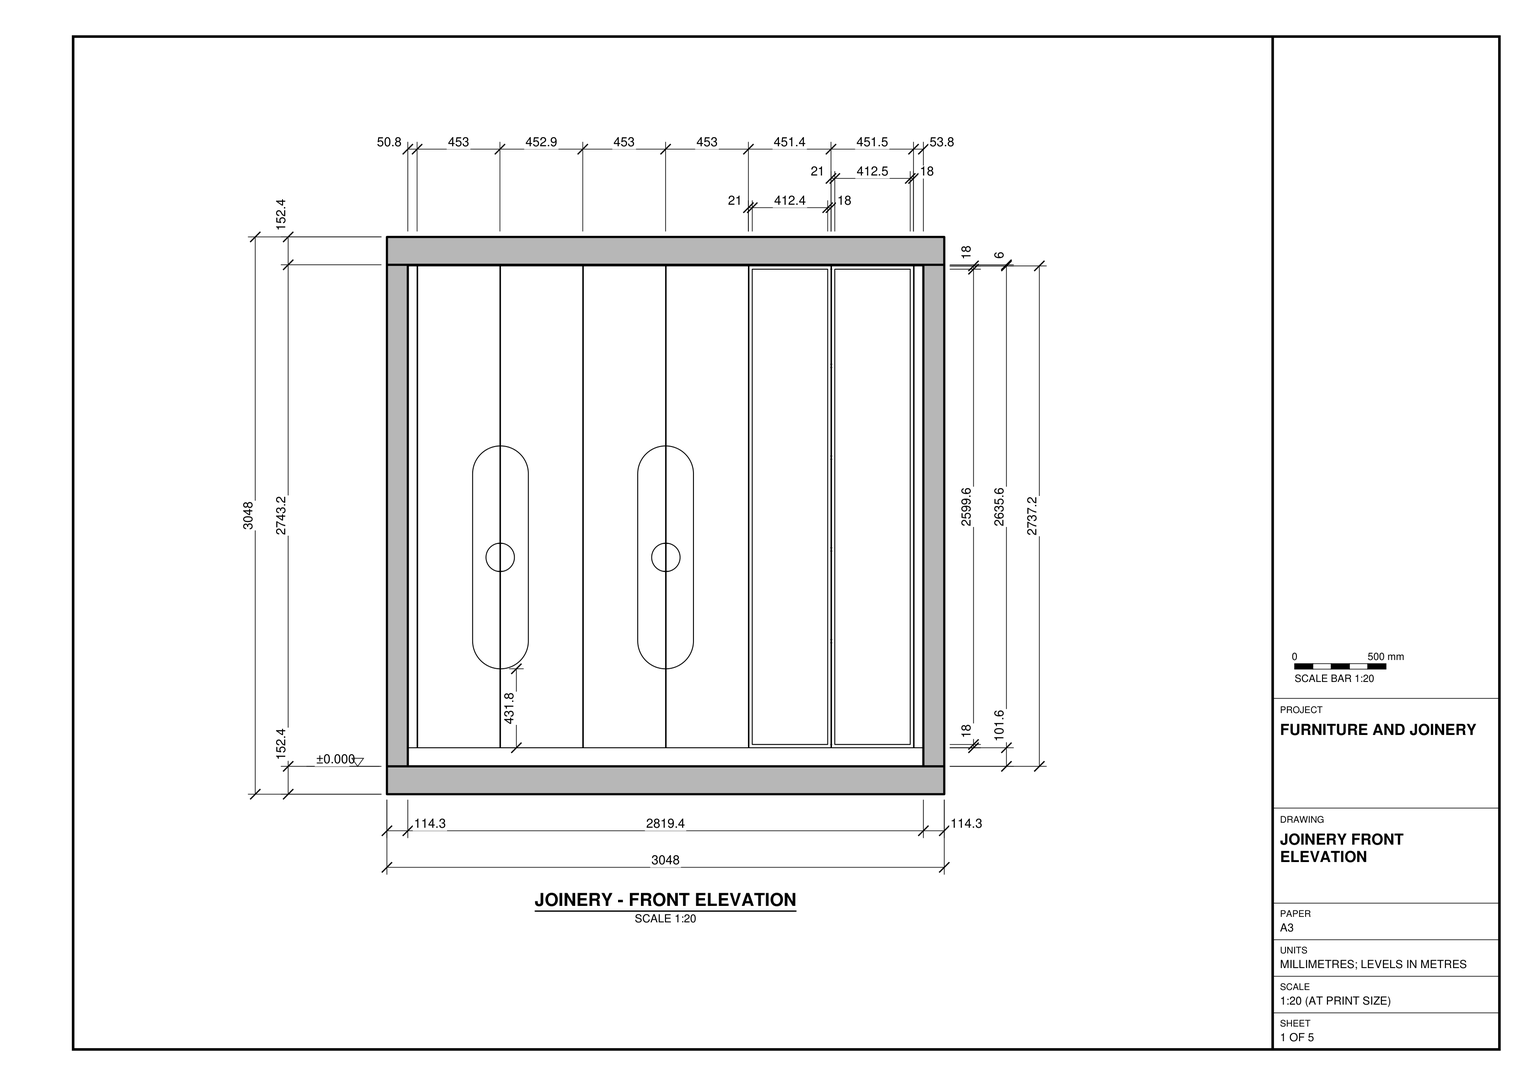
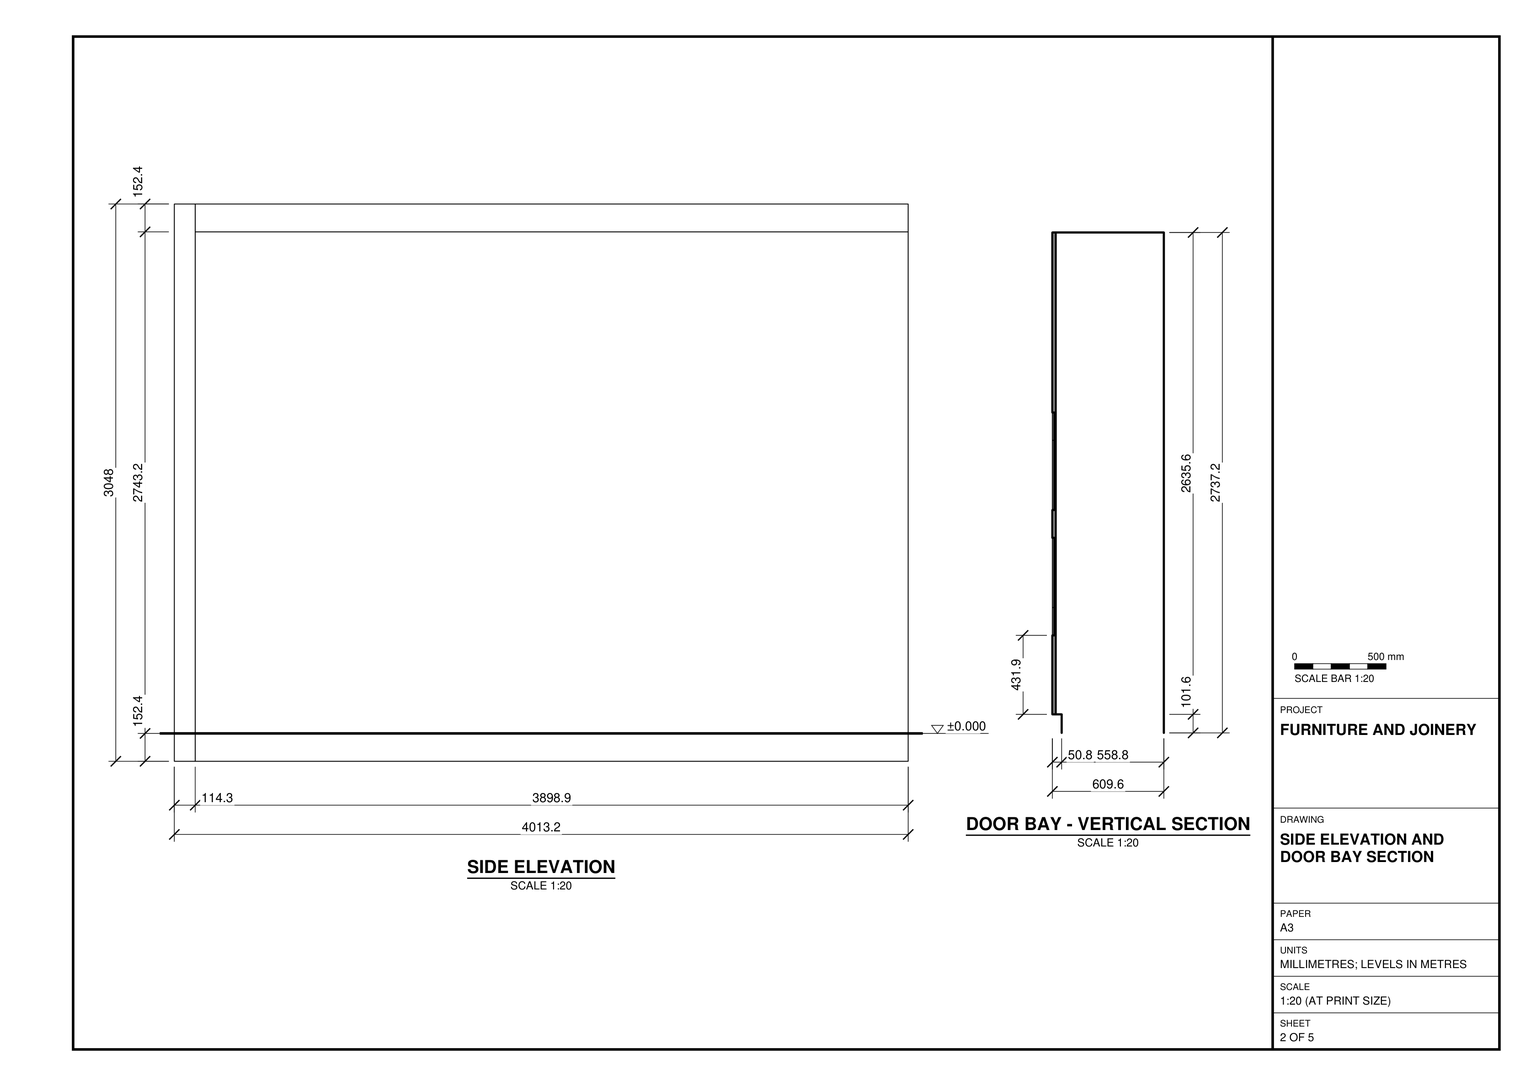
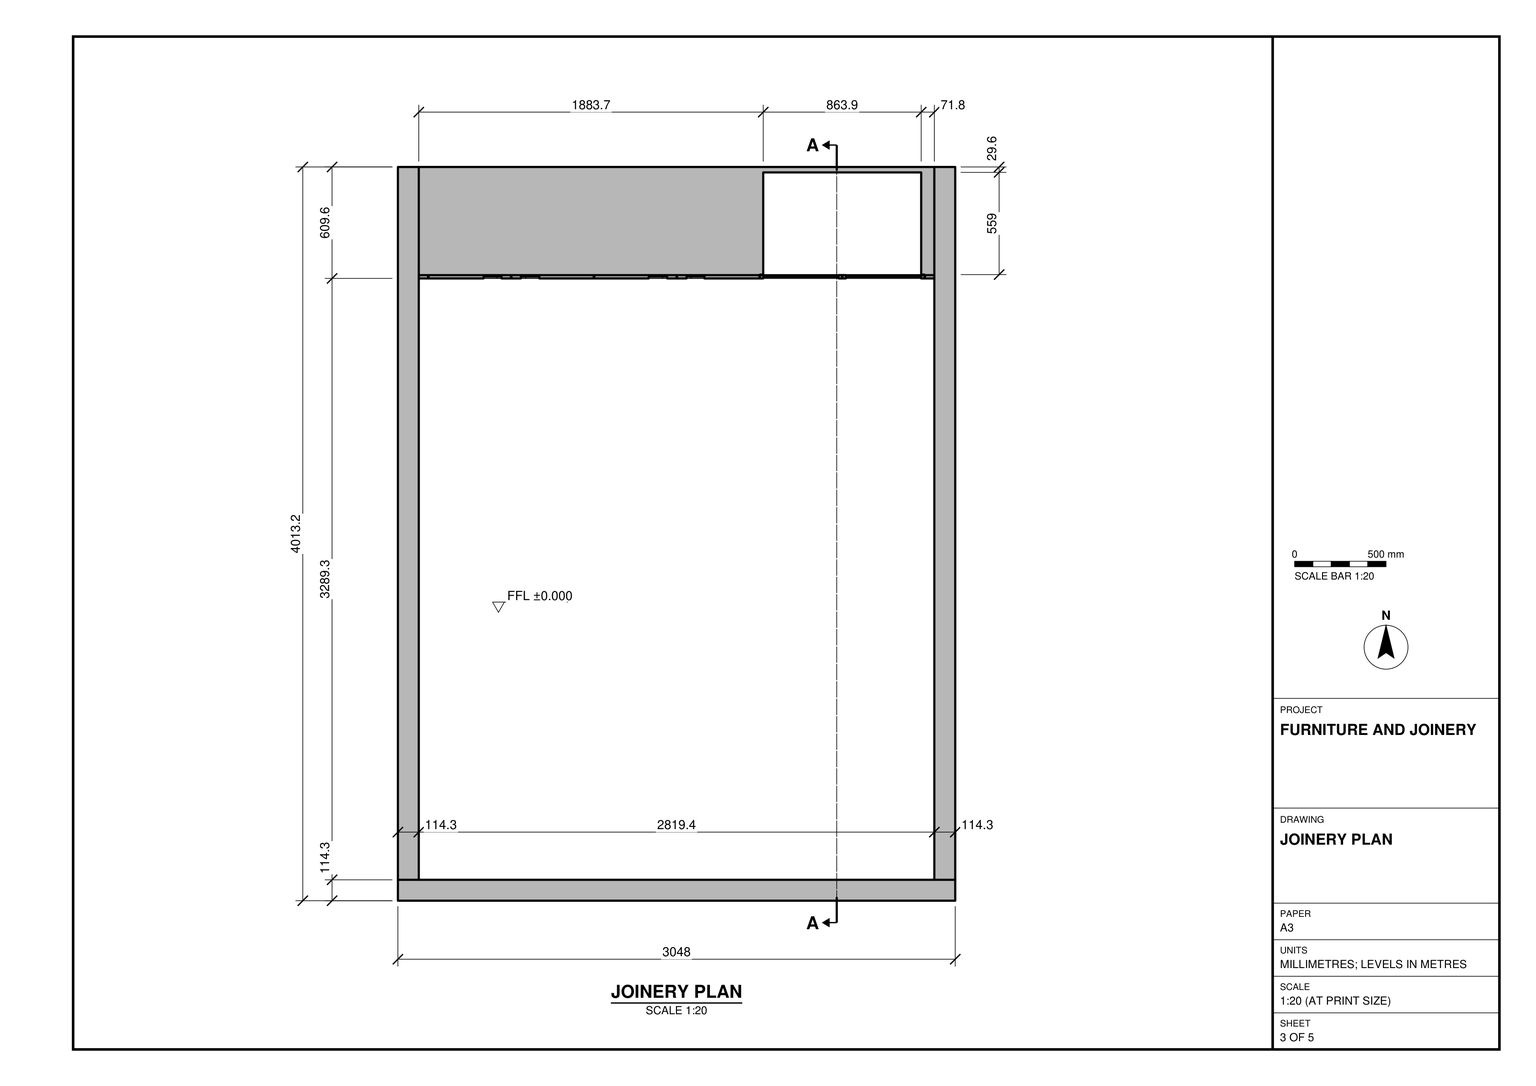
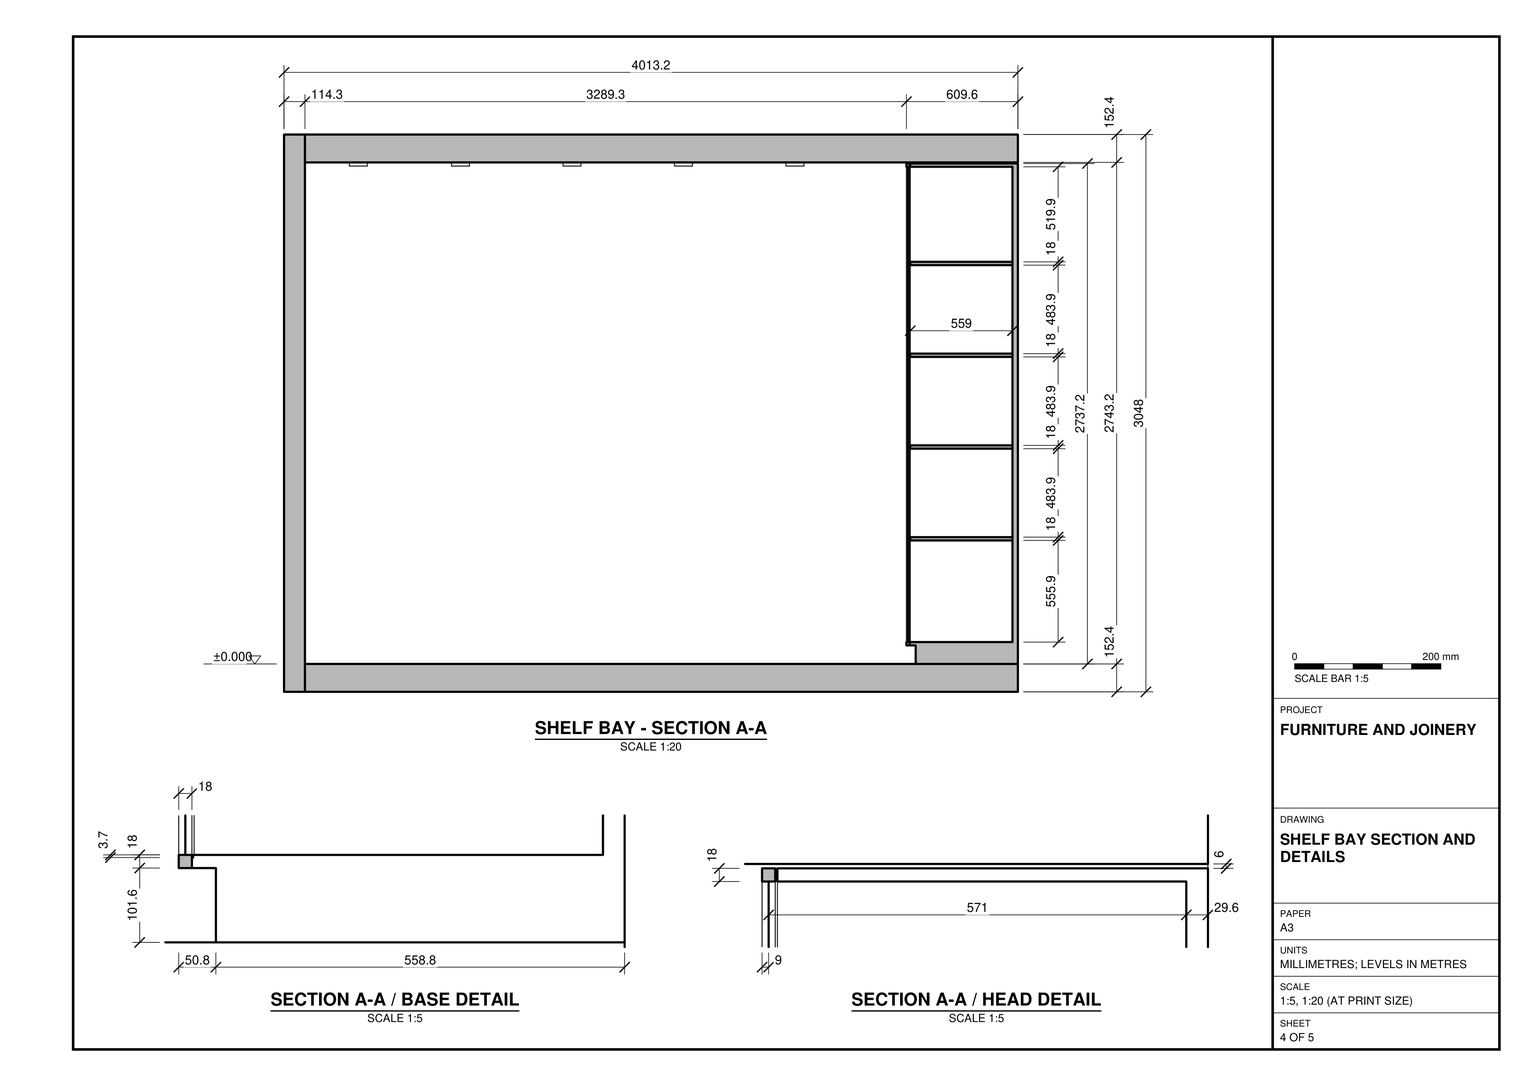
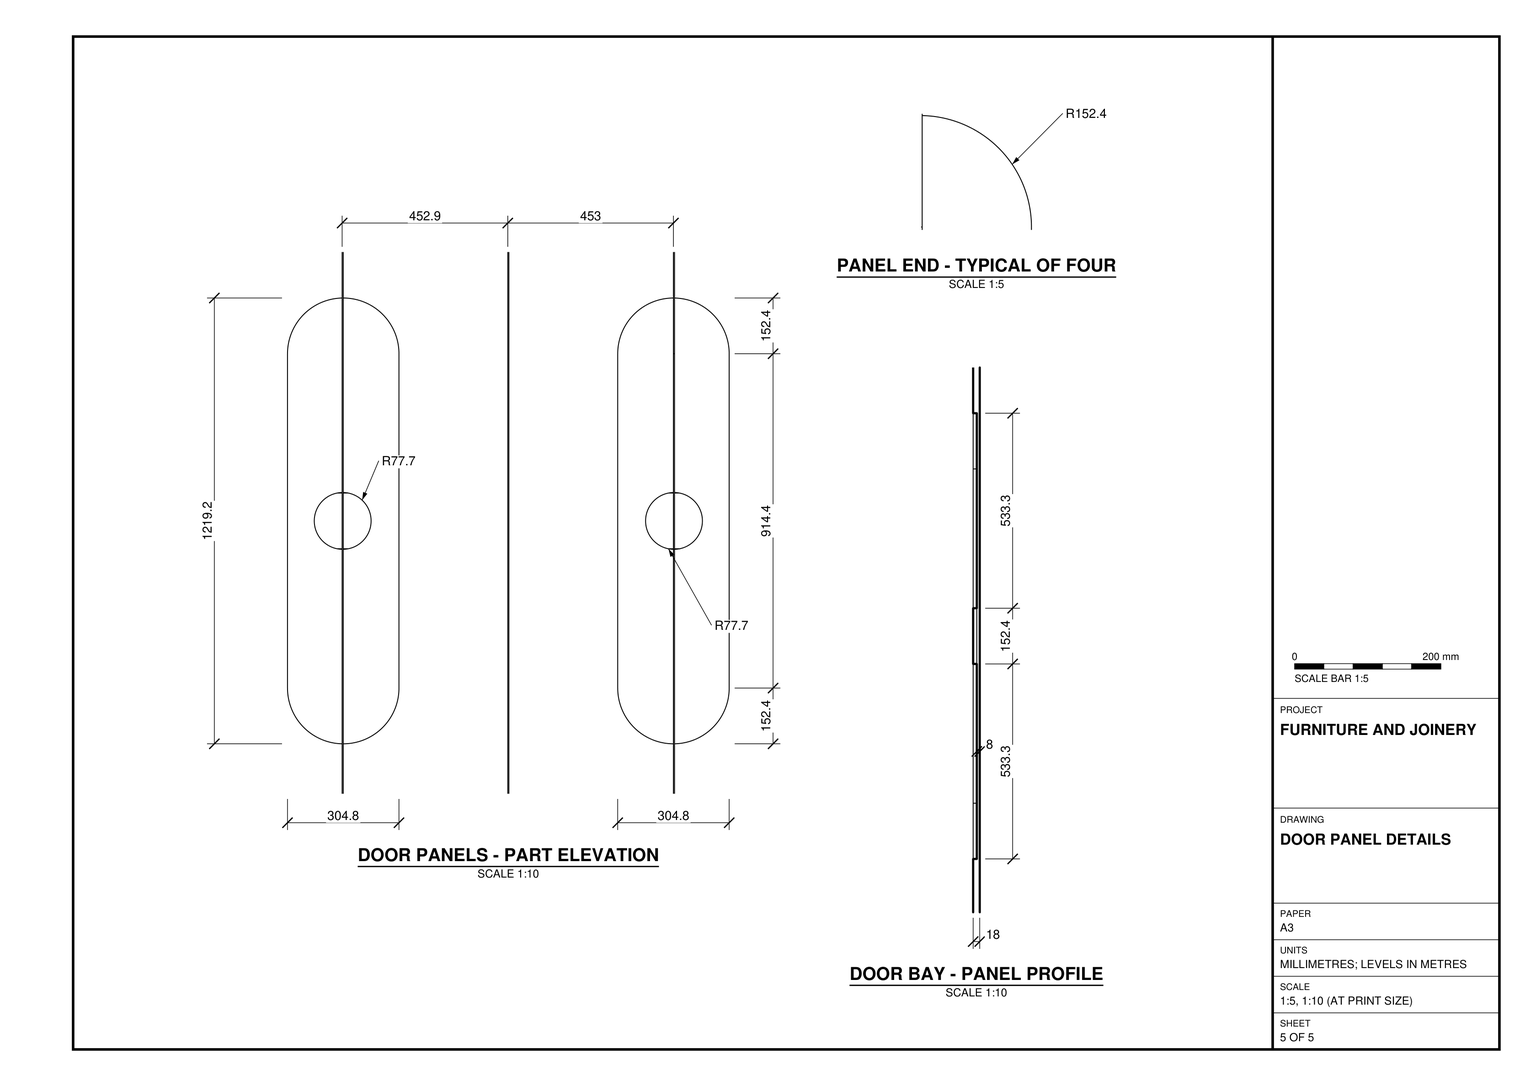
Build the wardrobe and its surrounding shell in SketchUp using task_files/diagram_01.pdf. Work in millimetres. The complete model is 3048 mm wide, 4013.2 mm deep and 3048 mm high. Set the finished floor at 0 mm, the ±0.000 datum shown on the sheets. Follow the plan for the wall layout. Use 114.3 mm walls and 152.4 mm floor and overhead slabs, leaving a clear height of 2743.2 mm.

Fit the wardrobe across the 2819.4 mm clear width at the end of the room shown in plan. Use the door-bay section to set its 609.6 mm depth and form the recessed plinth below the fronts. Follow the front elevation for the panel widths, narrow end fillers and clearance below the overhead slab. On the left, arrange four plain fronts as two pairs. Centre a tall, round-ended detail with a circular centre on the meeting line of each pair. On the right, frame the two tall rectangular panels with the narrow borders shown in elevation.

Keep the walls, slabs and built-in joinery as separate groups or components, and use components for repeated parts. Any decor or loose items shown may be suitable library components. Save one SketchUp model as output_files/six_panel_built_in_wardrobe_and_its_surrounding_shell.skp.

# SketchUp Ruby script. Lengths in millimetres.
U = 1.mm
M = Sketchup.active_model
def pt(a) = Geom::Point3d.new(a.map { |v| v * U })
def face(e, loops, mat)
  f = e.add_face(loops[0].map { |a| pt(a) })
  loops[1..].each { |l| e.add_face(l.map { |a| pt(a) }).erase! }
  f.material = f.back_material = mat if mat
  f
end
# faces: each face lists its corners as indices into pts; further lists are holes
def faces(e, pts, list, mat = nil) = list.each { |f| face(e, (f[0].is_a?(Array) ? f : [f]).map { |l| l.map { |i| pts[i] } }, mat) }
# xy, xz, yz: faces in a plane at the given z, y or x. An outline is a flat list of corners, or four numbers for a rectangle; further outlines are holes
def ring(l) = l.size == 4 ? [[l[0], l[1]], [l[2], l[1]], [l[2], l[3]], [l[0], l[3]]] : l.each_slice(2).to_a
def flat(e, list, mat, &to3) = list.each { |f| face(e, (f[0].is_a?(Array) ? f : [f]).map { |l| ring(l).map { |u, v| to3.(u, v) } }, mat) }
def xy(e, z, list, mat = nil) = flat(e, list, mat) { |x, y| [x, y, z] }
def xz(e, y, list, mat = nil) = flat(e, list, mat) { |x, z| [x, y, z] }
def yz(e, x, list, mat = nil) = flat(e, list, mat) { |y, z| [x, y, z] }
def lines(e, pts, list) = list.each { |a, b| e.add_line(pt(pts[a]), pt(pts[b])) }
# prism: a flat outline (further loops are holes) pulled along v
def prism(e, loops, v, mat = nil)
  f = face(e, loops, mat); d = Geom::Vector3d.new(v.map { |x| x * U })
  f.pushpull(f.normal.samedirection?(d) ? d.length : -d.length)
end
def box(e, o, s, mat = nil) = prism(e, [[o, [o[0] + s[0], o[1], o[2]], [o[0] + s[0], o[1] + s[1], o[2]], [o[0], o[1] + s[1], o[2]]]], [0, 0, s[2]], mat)
def at(x, y, z, deg = 0) = Geom::Transformation.translation(pt([x, y, z])) * Geom::Transformation.rotation(ORIGIN, Z_AXIS, deg.degrees)
def axes(o, x, y, z) = Geom::Transformation.new([*x, 0, *y, 0, *z, 0, *pt(o).to_a, 1])
def part(name) = M.definitions.add(name)
# library, detail: a bought-in or finely detailed component or shape, given as its bounding box
def library(name, o, s) = part(name).tap { |d| box(d.entities, o, s) }
def detail(e, o, s) = box(e.add_group.entities, o, s)
def put(e, d, t, mat = nil) = e.add_instance(d, t).tap { |i| i.material = mat if mat }
def group(e, t, mat = nil) = e.add_group.tap { |g| g.transformation = t; g.material = mat if mat }.entities
root = M.entities
c1 = library("Group\#3",[0,0,0],[2819.4,609.6,2737.2])
c2 = part("Group\#7")
xy(c2.entities,0,[[[49.2,0,36.5,1.7,24.6,6.6,14.4,14.4,6.6,24.6,1.7,36.5,0,49.2,1.7,61.9,6.6,73.8,14.4,84,24.6,91.8,36.5,96.7,49.2,98.4,61.9,96.7,73.8,91.8,84,84,91.8,73.8,96.7,61.9,98.4,49.2,96.7,36.5,91.8,24.6,84,14.4,73.8,6.6,61.9,1.7],[49.2,17.3,57.5,18.4,65.2,21.6,71.8,26.7,76.8,33.3,80,41,81.1,49.2,80,57.5,76.8,65.2,71.8,71.8,65.2,76.8,57.5,80,49.2,81.1,41,80,33.3,76.8,26.7,71.8,21.6,65.2,18.4,57.5,17.3,49.2,18.4,41,21.6,33.3,26.7,26.7,33.3,21.6,41,18.4]]])
xy(c2.entities,20,[[49.2,0,61.9,1.7,73.8,6.6,84,14.4,91.8,24.6,96.7,36.5,98.4,49.2,96.7,61.9,91.8,73.8,84,84,73.8,91.8,61.9,96.7,49.2,98.4,36.5,96.7,24.6,91.8,14.4,84,6.6,73.8,1.7,61.9,0,49.2,1.7,36.5,6.6,24.6,14.4,14.4,24.6,6.6,36.5,1.7]])
p = [[49.2,0,20],[36.5,1.7,20],[36.5,1.7,0],[49.2,0,0],[61.9,1.7,20],[61.9,1.7,0],
  [24.6,6.6,20],[24.6,6.6,0],[73.8,6.6,20],[73.8,6.6,0],[14.4,14.4,20],[14.4,14.4,0],
  [84,14.4,20],[84,14.4,0],[6.6,24.6,20],[6.6,24.6,0],[91.8,24.6,20],[91.8,24.6,0],
  [49.2,17.3,0],[41,18.4,0],[41,18.4,10],[49.2,17.3,10],[57.5,18.4,0],[57.5,18.4,10],
  [33.3,21.6,0],[33.3,21.6,10],[65.2,21.6,0],[65.2,21.6,10],[26.7,26.7,0],[26.7,26.7,10],
  [71.8,26.7,0],[71.8,26.7,10],[1.7,36.5,20],[1.7,36.5,0],[96.7,36.5,20],[96.7,36.5,0],
  [21.6,33.3,0],[21.6,33.3,10],[76.8,33.3,0],[76.8,33.3,10],[18.4,41,0],[18.4,41,10],
  [80,41,0],[80,41,10],[0,49.2,20],[0,49.2,0],[98.4,49.2,20],[98.4,49.2,0],
  [17.3,49.2,0],[17.3,49.2,10],[81.1,49.2,0],[81.1,49.2,10],[1.7,61.9,20],[1.7,61.9,0],
  [18.4,57.5,0],[18.4,57.5,10],[80,57.5,0],[80,57.5,10],[96.7,61.9,20],[96.7,61.9,0],
  [21.6,65.2,0],[21.6,65.2,10],[76.8,65.2,0],[76.8,65.2,10],[6.6,73.8,20],[6.6,73.8,0],
  [91.8,73.8,20],[91.8,73.8,0],[26.7,71.8,0],[26.7,71.8,10],[71.8,71.8,0],[71.8,71.8,10],
  [33.3,76.8,0],[33.3,76.8,10],[65.2,76.8,0],[65.2,76.8,10],[14.4,84,20],[14.4,84,0],
  [84,84,20],[84,84,0],[41,80,0],[41,80,10],[57.5,80,0],[57.5,80,10],
  [49.2,81.1,0],[49.2,81.1,10],[24.6,91.8,20],[24.6,91.8,0],[73.8,91.8,20],[73.8,91.8,0],
  [36.5,96.7,20],[36.5,96.7,0],[61.9,96.7,20],[61.9,96.7,0],[49.2,98.4,20],[49.2,98.4,0]]
faces(c2.entities,p,[[0,1,2,3],[4,0,3,5],[1,6,7,2],[8,4,5,9],[6,10,11,7],[12,8,9,13],[10,14,15,11],[16,12,13,17],
  [18,19,20,21],[22,18,21,23],[19,24,25,20],[26,22,23,27],[24,28,29,25],[30,26,27,31],[14,32,33,15],[34,16,17,35],
  [28,36,37,29],[38,30,31,39],[36,40,41,37],[42,38,39,43],[32,44,45,33],[46,34,35,47],[40,48,49,41],[50,42,43,51],
  [44,52,53,45],[48,54,55,49],[56,50,51,57],[58,46,47,59],[54,60,61,55],[62,56,57,63],[52,64,65,53],[66,58,59,67],
  [60,68,69,61],[70,62,63,71],[68,72,73,69],[74,70,71,75],[64,76,77,65],[78,66,67,79],[72,80,81,73],[82,74,75,83],
  [80,84,85,81],[84,82,83,85],[76,86,87,77],[88,78,79,89],[86,90,91,87],[92,88,89,93],[90,94,95,91],[94,92,93,95]])
g1 = group(root,at(0,965.2,0))
xy(g1,0,[[0,-965.2,3048,-850.9],[0,-850.9,3048,3048]])
xy(g1,152.4,[[0,-850.9,3048,3048]])
xy(g1,3048,[[0,-965.2,3048,-850.9]])
xz(g1,-965.2,[[0,0,3048,3048]])
xz(g1,-850.9,[[0,0,3048,152.4],[0,152.4,3048,3048]])
xz(g1,3048,[[0,0,3048,152.4]])
yz(g1,0,[[-965.2,0,-850.9,3048],[-850.9,0,3048,152.4]])
yz(g1,3048,[[-965.2,0,-850.9,3048],[-850.9,0,3048,152.4]])
g2 = group(root,at(0,965.2,152.4))
box(g2,[0,-850.9,0],[114.3,3898.9,2743.2])
g3 = group(root,at(2933.7,965.2,152.4))
box(g3,[0,-850.9,0],[114.3,3898.9,2743.2])
put(root,c1,at(114.3,3403.6,152.4))
g4 = group(root,at(0,965.2,2895.6))
xy(g4,0,[[[0,-850.9,3048,3048],[741.2,-420.1,2265.2,1697.6]],[766.6,-394.7,2239.8,1672.2]])
xy(g4,152.4,[[0,-850.9,3048,3048]])
xz(g4,-850.9,[[0,0,3048,152.4]])
xz(g4,3048,[[0,0,3048,152.4]])
yz(g4,0,[[-850.9,0,3048,152.4]])
yz(g4,3048,[[-850.9,0,3048,152.4]])
g5 = group(g4,at(741.2,-420.1,0))
xy(g5,0,[[[0,0,1524,2117.7],[25.4,25.4,1498.6,2092.3]]])
g6 = group(root,at(582.2,2762.1,2885.6))
xy(g6,0,[[31.9,0,23.6,1.1,15.9,4.3,9.3,9.3,4.3,15.9,1.1,23.6,0,31.9,1.1,40.1,4.3,47.8,9.3,54.4,15.9,59.5,23.6,62.7,31.9,63.8,40.1,62.7,47.8,59.5,54.4,54.4,59.5,47.8,62.7,40.1,63.8,31.9,62.7,23.6,59.5,15.9,54.4,9.3,47.8,4.3,40.1,1.1]])
put(root,c2,at(564.9,2744.8,2875.6))
put(root,c2,at(1495.1,2744.8,2875.6))
put(root,c2,at(2522.2,2744.8,2875.6))
put(root,c2,at(2522.2,2135.2,2875.6))
put(root,c2,at(564.9,2135.2,2875.6))
put(root,c2,at(2522.2,1525.6,2875.6))
put(root,c2,at(564.9,1525.6,2875.6))
put(root,c2,at(2522.2,916,2875.6))
put(root,c2,at(564.9,916,2875.6))
put(root,c2,at(2522.2,357.2,2875.6))
put(root,c2,at(1495.1,357.2,2875.6))
put(root,c2,at(564.9,357.2,2875.6))
